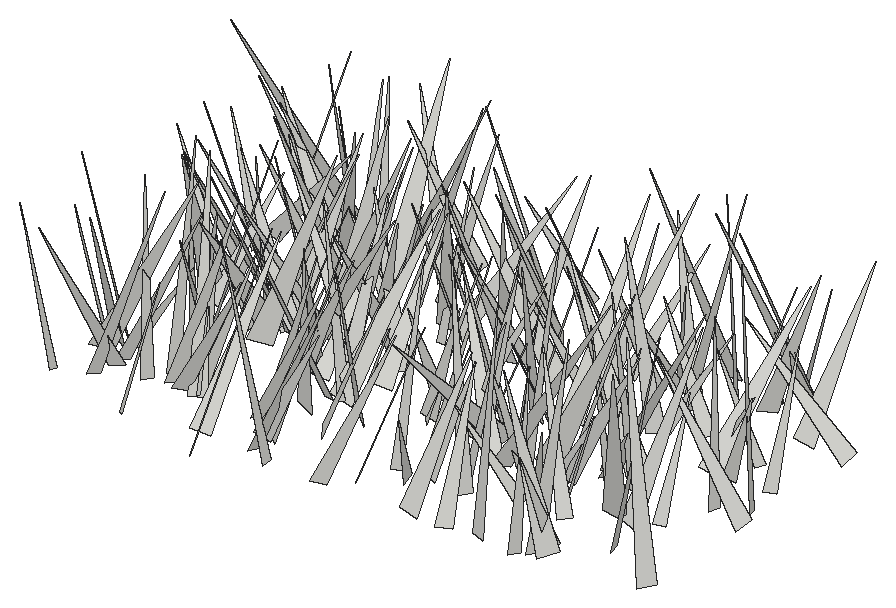
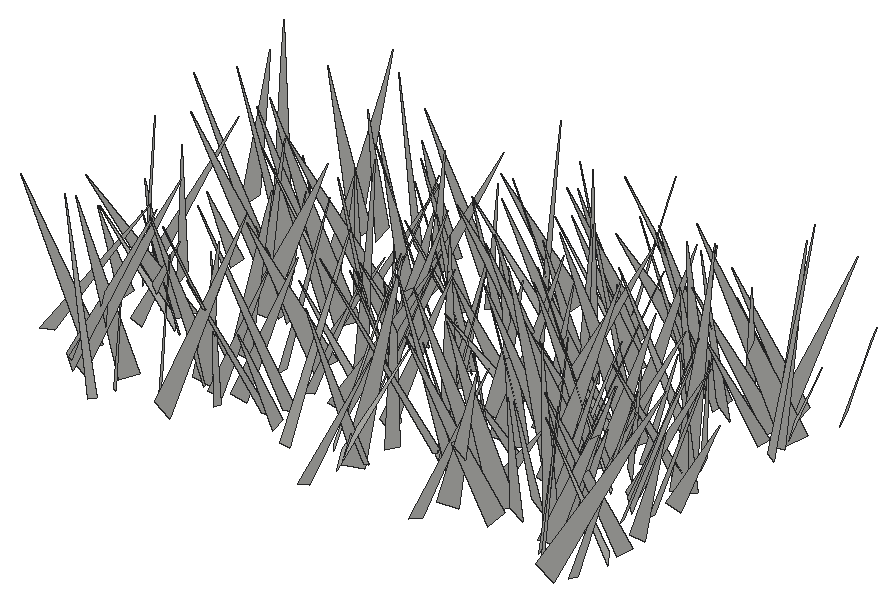
# SketchUp Ruby script. Lengths in inches.
U = 1.inch
M = Sketchup.active_model
def pt(a) = Geom::Point3d.new(a.map { |v| v * U })
def face(e, loops, mat)
  f = e.add_face(loops[0].map { |a| pt(a) })
  loops[1..].each { |l| e.add_face(l.map { |a| pt(a) }).erase! }
  f.material = f.back_material = mat if mat
  f
end
# faces: each face lists its corners as indices into pts; further lists are holes
def faces(e, pts, list, mat = nil) = list.each { |f| face(e, (f[0].is_a?(Array) ? f : [f]).map { |l| l.map { |i| pts[i] } }, mat) }
# xy, xz, yz: faces in a plane at the given z, y or x. An outline is a flat list of corners, or four numbers for a rectangle; further outlines are holes
def ring(l) = l.size == 4 ? [[l[0], l[1]], [l[2], l[1]], [l[2], l[3]], [l[0], l[3]]] : l.each_slice(2).to_a
def flat(e, list, mat, &to3) = list.each { |f| face(e, (f[0].is_a?(Array) ? f : [f]).map { |l| ring(l).map { |u, v| to3.(u, v) } }, mat) }
def xy(e, z, list, mat = nil) = flat(e, list, mat) { |x, y| [x, y, z] }
def xz(e, y, list, mat = nil) = flat(e, list, mat) { |x, z| [x, y, z] }
def yz(e, x, list, mat = nil) = flat(e, list, mat) { |y, z| [x, y, z] }
def lines(e, pts, list) = list.each { |a, b| e.add_line(pt(pts[a]), pt(pts[b])) }
# prism: a flat outline (further loops are holes) pulled along v
def prism(e, loops, v, mat = nil)
  f = face(e, loops, mat); d = Geom::Vector3d.new(v.map { |x| x * U })
  f.pushpull(f.normal.samedirection?(d) ? d.length : -d.length)
end
def box(e, o, s, mat = nil) = prism(e, [[o, [o[0] + s[0], o[1], o[2]], [o[0] + s[0], o[1] + s[1], o[2]], [o[0], o[1] + s[1], o[2]]]], [0, 0, s[2]], mat)
def at(x, y, z, deg = 0) = Geom::Transformation.translation(pt([x, y, z])) * Geom::Transformation.rotation(ORIGIN, Z_AXIS, deg.degrees)
def axes(o, x, y, z) = Geom::Transformation.new([*x, 0, *y, 0, *z, 0, *pt(o).to_a, 1])
def part(name) = M.definitions.add(name)
# library, detail: a bought-in or finely detailed component or shape, given as its bounding box
def library(name, o, s) = part(name).tap { |d| box(d.entities, o, s) }
def detail(e, o, s) = box(e.add_group.entities, o, s)
def put(e, d, t, mat = nil) = e.add_instance(d, t).tap { |i| i.material = mat if mat }
def group(e, t, mat = nil) = e.add_group.tap { |g| g.transformation = t; g.material = mat if mat }.entities
root = M.entities
c1 = part("fur_instance\#9")
p = [[0.8125,0,1.79],[0.67,-0.02,1.48],[0,-0.11,0],[0,0.11,0]]
faces(c1.entities,p,[[0,1,2,3]])
put(root,c1,axes([495.01,358.53,-21.66],[4.68158,-4.31782,3.21331],[-4.18207,-5.59908,-1.43065],[-3.3881,0.94493,6.20597]))
put(root,c1,axes([494.79,359.46,-21.66],[4.08531,-1.79648,1.28746],[-1.24322,-4.1049,-1.78292],[-1.82737,-1.22355,4.09124]))
put(root,c1,axes([473.0625,356.67,-21.66],[-7.26619,-2.16018,0.91047],[-2.32448,7.02333,-1.88745],[0.30351,2.07347,7.34176]))
put(root,c1,axes([468.41,354.61,-21.66],[6.47169,4.71895,0.84374],[4.29058,-6.33416,2.51645],[-2.13805,1.57262,7.60387]))
put(root,c1,axes([461.51,355.93,-21.66],[2.88186,3.44939,0.31018],[3.15851,-2.7832,1.60537],[-1.42067,0.8094,4.19835]))
put(root,c1,axes([457.41,360.6875,-21.66],[0.6668,-6.36542,0.43774],[-6.10772,-0.7641,-1.80742],[-1.84553,0.22889,6.13974]))
put(root,c1,axes([484.39,357.22,-21.66],[0.24671,6.36494,1.6516],[6.30189,0.24313,-1.87833],[1.87786,-1.65213,6.08648]))
put(root,c1,axes([477.34,356.72,-21.66],[5.30796,-1.91017,1.71118],[-2.50762,-4.68997,2.54311],[-0.53734,3.01775,5.03546]))
put(root,c1,axes([470.7,359.16,-21.66],[2.62599,-5.06265,0.78885],[-4.77605,-2.09765,2.43674],[1.85526,1.76578,5.15641]))
put(root,c1,axes([481.65,360.63,-21.66],[4.12034,-0.14152,0.59374],[0.17297,-3.61498,-2.06197],[-0.58535,-2.06437,3.57009]))
put(root,c1,axes([487.48,357.11,-21.66],[-4.32625,3.6169,1.13686],[3.35652,4.45591,-1.40339],[1.76301,0.39209,5.46158]))
put(root,c1,axes([454.46,357.73,-21.66],[-5.41168,-1.42657,0.35166],[-1.45652,5.03228,-1.99993],[-0.1932,2.0214,5.22701]))
put(root,c1,axes([493.19,357.29,-21.66],[-6.05732,0.47074,1.68041],[-0.07648,5.99257,-1.95441],[1.74342,1.89841,5.75265]))
put(root,c1,axes([471.32,357.58,-21.66],[6.28882,0.29269,0.74734],[0.08478,-6.11246,1.68051],[-0.79813,1.65699,6.06719]))
put(root,c1,axes([489.93,357.61,-21.66],[3.45024,7.01244,2.07893],[6.95776,-3.8555,1.45774],[-2.25516,-1.1667,7.67811]))
put(root,c1,axes([494.21,358.21,-21.66],[-6.74927,1.80081,2.69667],[1.18797,7.16726,-1.81295],[3.01723,1.2063,6.74602]))
put(root,c1,axes([462.65,360.75,-21.66],[4.53332,-3.78068,0.06575],[-3.6354,-4.32956,1.69931],[1.04008,1.34544,5.65304]))
put(root,c1,axes([455.38,363.32,-21.66],[-1.80775,-6.68688,0.47497],[-6.40102,1.86794,1.93536],[1.9917,-0.06601,6.65106]))
put(root,c1,axes([467.12,357.18,-21.66],[-4.67484,5.38464,0.57126],[4.73589,4.43174,-3.01759],[2.62527,1.59378,6.46085]))
put(root,c1,axes([479.14,358.47,-21.66],[4.7893,3.01055,0.30481],[2.77693,-4.59952,1.79634],[-1.20208,1.36921,5.36414]))
put(root,c1,axes([489.45,362.83,-21.66],[-4.59032,-0.23962,0.17171],[-0.16134,4.28449,1.66587],[0.24672,-1.65642,4.28408]))
put(root,c1,axes([456.87,358.93,-21.66],[6.5419,0.41912,1.71437],[-0.23349,-6.31856,2.43568],[-1.74935,2.41069,6.08602]))
put(root,c1,axes([502.66,359.23,-21.66],[-8.1921,1.36867,0.61461],[1.20152,8.02801,-1.8625],[0.89853,1.74336,8.09413]))
put(root,c1,axes([463.77,361.33,-21.66],[3.63408,5.21962,1.38175],[5.32326,-3.18476,-1.96987],[0.90365,-2.23003,6.04736]))
put(root,c1,axes([468.93,361.03,-21.66],[5.6454,-1.61471,0.55375],[-1.70236,-5.46688,1.41409],[-0.12614,1.5134,5.69896]))
put(root,c1,axes([482.48,361.83,-21.66],[0.05129,-4.93553,2.34933],[-4.99892,0.90807,2.01684],[2.21125,2.16734,4.50493]))
put(root,c1,axes([468.37,363.05,-21.66],[5.01746,5.30698,2.27397],[5.71554,-4.13917,-2.95123],[0.81705,-3.63499,6.68051]))
put(root,c1,axes([473.91,365.3125,-21.66],[-3.7888,-7.35051,1.42507],[-6.56657,4.02946,3.32556],[3.59735,-0.38635,7.57137]))
put(root,c1,axes([471.67,359.15,-21.66],[4.6203,4.92142,0.32663],[4.69042,-4.52255,1.79463],[-1.52544,1.00021,6.50745]))
put(root,c1,axes([473.32,362.11,-21.66],[5.31801,3.62577,0.57345],[3.65614,-5.14142,-1.39812],[0.32822,-1.47507,6.28273]))
put(root,c1,axes([454.96,364.62,-21.66],[-4.90749,-6.3294,1.61985],[-6.13533,5.16095,1.5783],[2.24565,0.26836,7.85199]))
put(root,c1,axes([495.2,365.25,-21.66],[1.43301,-8.2393,0.15598],[-8.02359,-1.35888,1.93375],[1.87948,0.48092,8.13635]))
put(root,c1,axes([461.71,361.26,-21.66],[6.69974,-1.69034,1.74311],[-2.11177,-6.58131,1.73465],[-1.19837,2.1474,6.68841]))
put(root,c1,axes([470.45,363.9,-21.66],[-1.45623,-6.82166,1.9418],[-6.84757,1.86878,1.42991],[1.84835,1.54881,6.82723]))
put(root,c1,axes([460.1,360.48,-21.66],[-6.71472,0.14595,1.05093],[-0.21339,6.41005,-2.25365],[1.03933,2.25902,6.32691]))
put(root,c1,axes([455.04,361.94,-21.66],[6.5519,-4.81181,0.9912],[-4.80718,-5.93833,2.94799],[1.01342,2.94042,7.57563]))
put(root,c1,axes([464.29,361.04,-21.66],[-5.1152,1.11044,1.16629],[0.73583,5.06638,-1.59654],[1.43244,1.36283,4.98492]))
put(root,c1,axes([489.3,364.63,-21.66],[-0.15941,-4.26775,0.08772],[-3.87813,0.18147,1.78158],[1.78369,0.01316,3.88138]))
put(root,c1,axes([455.64,362.03,-21.66],[-4.45593,-2.02584,0.38216],[-1.95722,3.87117,-2.29973],[-0.64758,2.23951,4.32095]))
put(root,c1,axes([460.95,366,-21.66],[-1.84691,-6.18778,0.26193],[-5.9057,1.84189,1.87043],[1.86547,-0.29517,6.18071]))
put(root,c1,axes([464.13,360.71,-21.66],[0.27633,8.1596,0.76138],[7.93766,-0.45592,2.00518],[-2.0377,-0.66947,7.91421]))
put(root,c1,axes([457.15,361.625,-21.66],[6.04009,-0.71684,0.90558],[-1.00409,-5.64184,2.23115],[-0.57074,2.3393,5.65849]))
put(root,c1,axes([485.76,361.42,-21.66],[-7.72963,0.57294,0.92033],[0.30078,7.49944,-2.14251],[1.04153,2.08628,7.44883]))
put(root,c1,axes([497.92,361.75,-21.66],[6.4621,3.38539,1.99868],[3.00841,-6.73382,1.67909],[-2.53082,0.63956,7.09931]))
put(root,c1,axes([483.41,368.64,-21.66],[5.32765,-5.22538,0.29084],[-4.03169,-4.36253,-4.52625],[-3.33686,-3.07194,5.93309]))
put(root,c1,axes([456.56,363.36,-21.66],[3.29977,-2.51906,0.3221],[-2.3698,-2.86445,1.87534],[0.91296,1.66948,3.70368]))
put(root,c1,axes([480.27,361.18,-21.66],[2.16067,6.65454,0.44246],[6.23565,-2.18071,2.34697],[-2.36543,0.32979,6.59114]))
put(root,c1,axes([461.14,361.86,-21.66],[2.8075,7.47142,1.47372],[7.21104,-3.11318,2.04573],[-2.44844,-0.60171,7.71486]))
put(root,c1,axes([491.26,365.27,-21.66],[3.99613,2.0991,0.80323],[2.24013,-3.58697,-1.77087],[0.18236,-1.93595,4.15203]))
put(root,c1,axes([492.84,362.98,-21.66],[-1.19348,5.65379,0.3473],[5.3271,0.99964,2.033],[-1.92561,-0.73875,5.40894]))
put(root,c1,axes([470.83,365.9,-21.66],[-3.56669,-5.90918,0.59479],[-5.71236,3.22345,-2.22975],[-1.62517,1.63841,6.53207]))
put(root,c1,axes([484.51,363.29,-21.66],[4.61652,6.22378,1.13894],[6.03614,-4.75491,1.51682],[-1.89675,0.0163,7.59914]))
put(root,c1,axes([480.61,363.97,-21.66],[3.00596,2.69315,0.13963],[2.45938,-2.82346,1.51258],[-1.10635,1.04086,3.74179]))
put(root,c1,axes([467.49,368.98,-21.66],[-1.30326,-6.4856,0.41929],[-6.05179,1.36694,2.33336],[2.36951,-0.07596,6.19006]))
put(root,c1,axes([462.64,370.46,-21.66],[6.08431,-4.17162,0.61258],[-3.3903,-5.47976,-3.64343],[-2.50671,-2.71408,6.41457]))
put(root,c1,axes([472.63,367.23,-21.66],[3.70621,1.73352,0.50221],[1.78343,-3.34171,-1.62653],[0.27688,-1.67963,3.75439]))
put(root,c1,axes([489.52,367.13,-21.66],[2.95462,-6.48005,1.02046],[-5.97059,-2.19282,3.36242],[2.71745,2.2277,6.27814]))
put(root,c1,axes([496.72,364.875,-21.66],[1.72672,7.47142,1.23195],[7.48463,-1.49226,-1.44043],[1.14896,-1.50745,7.53186]))
put(root,c1,axes([467.25,367.52,-21.66],[3.81653,-4.78014,0.36891],[-4.62204,-3.54318,1.90641],[1.2738,1.46558,5.81217]))
put(root,c1,axes([482,367.45,-21.66],[1.0853,-7.02468,2.48253],[-7.23303,-0.3918,2.05344],[1.78669,2.68091,6.80495]))
put(root,c1,axes([486.08,366.82,-21.66],[-6.99068,-2.50094,0.47101],[-2.54423,6.83653,-1.46112],[-0.05835,1.53405,7.27938]))
put(root,c1,axes([477.54,367.91,-21.66],[1.22983,-5.08709,1.30795],[-5.046,-0.77126,1.74491],[1.45845,1.62123,4.93419]))
put(root,c1,axes([485.17,365.87,-21.66],[7.21653,-2.33327,0.39687],[-2.31249,-6.67999,2.77668],[0.50399,2.75925,7.05779]))
put(root,c1,axes([480.72,363.98,-21.66],[4.07419,5.57288,0.07978],[5.18286,-3.82462,2.48447],[-2.04971,1.40628,6.44076]))
put(root,c1,axes([484.37,366.11,-21.66],[-3.04335,5.85133,0.32291],[5.70958,2.87864,1.64877],[-1.32023,-1.03909,6.38604]))
put(root,c1,axes([487.54,367.96,-21.66],[4.40599,-6.63506,1.39046],[-6.52465,-3.70025,3.01783],[1.84021,2.76664,7.37085]))
put(root,c1,axes([466.51,368.04,-21.66],[6.17977,-5.38552,0.13557],[-5.06059,-5.73249,2.95646],[1.84733,2.31224,7.64543]))
put(root,c1,axes([477.4,367.84,-21.66],[5.01329,4.55618,1.17415],[4.70331,-4.80639,-1.43108],[0.12753,-1.84671,6.62147]))
put(root,c1,axes([471.96,366.15,-21.66],[-6.70082,0.16595,0.10129],[0.12128,6.29761,-2.29436],[0.15195,2.29157,6.29797]))
put(root,c1,axes([490.59,365.47,-21.66],[4.99959,5.18328,0.38062],[5.01525,-4.9501,1.53324],[-1.36326,0.79826,7.03643]))
put(root,c1,axes([498.22,366.13,-21.66],[-3.90191,2.21296,0.38649],[1.88444,3.64598,-1.85127],[1.22289,1.44261,4.08594]))
put(root,c1,axes([456.65,371.74,-21.66],[7.11754,-4.23376,0.53848],[-3.90576,-6.88369,-2.49681],[-1.7204,-1.88792,7.89621]))
put(root,c1,axes([471.64,366.18,-21.66],[-0.75445,7.6495,1.46212],[7.18414,1.25072,-2.83648],[3.00677,-1.06897,7.14412]))
put(root,c1,axes([502.54,369.54,-21.66],[-6.59727,0.97904,0.29915],[1.02311,6.37288,1.70633],[0.03533,-1.73199,6.44755]))
put(root,c1,axes([476.84,370.16,-21.66],[3.36953,-3.09183,0.80409],[-2.80421,-3.42236,-1.4084],[-1.53048,-0.53643,4.35081]))
put(root,c1,axes([493.36,367.04,-21.66],[-5.59441,-0.96055,0.72122],[-1.15543,5.24244,-1.98041],[0.32833,2.08191,5.31959]))
put(root,c1,axes([460.2,366.45,-21.66],[6.70956,3.50603,1.11128],[3.28027,-6.75003,1.49074],[-1.66343,0.8308,7.42214]))
put(root,c1,axes([460.97,370.38,-21.66],[-3.68775,-0.43694,1.2324],[0.03671,3.65173,1.40455],[1.30705,-1.33536,3.43768]))
put(root,c1,axes([494.14,368.64,-21.66],[1.80379,6.11401,2.80003],[6.29213,-2.55743,1.53087],[-2.37284,-2.13386,6.18799]))
put(root,c1,axes([486.97,366.5,-21.66],[3.53249,6.50702,1.2231],[6.07163,-3.73652,2.34297],[-2.64057,0.11331,7.02355]))
put(root,c1,axes([487.37,369.79,-21.66],[-2.45268,-3.25533,0.28731],[-3.08329,2.18606,-1.55237],[-1.08306,1.14864,3.76868]))
put(root,c1,axes([457.76,368.17,-21.66],[-5.24858,-0.93793,1.2858],[-1.33069,5.01688,-1.77222],[0.87308,2.00792,5.02857]))
put(root,c1,axes([482.15,367.73,-21.66],[3.84867,2.11329,0.22175],[1.92609,-3.66331,1.48248],[-0.8974,1.20066,4.13285]))
put(root,c1,axes([482.04,370.46,-21.66],[-2.37076,-5.83706,1.32394],[-5.9146,2.06646,-1.48049],[-0.91737,1.76156,6.12372]))
put(root,c1,axes([462.75,368.8125,-21.66],[5.54256,-5.39998,2.31392],[-5.86744,-4.92827,2.55329],[0.29519,3.43313,7.30483]))
put(root,c1,axes([464.42,373.07,-21.66],[-5.86145,-3.99032,0.23805],[-3.68658,5.55942,2.41617],[1.54546,-1.87245,6.66644]))
put(root,c1,axes([468.73,367.71,-21.66],[-1.68385,4.77561,0.18208],[4.53538,1.65768,-1.53538],[1.50664,0.34725,4.82539]))
put(root,c1,axes([456.03,371.4,-21.66],[-0.42992,-4.68733,0.89248],[-4.33891,0.75688,1.88505],[1.98531,0.63912,4.31306]))
put(root,c1,axes([491.55,369.12,-21.66],[7.5928,-1.32868,0.07278],[-1.31152,-7.40102,1.71058],[0.22497,1.69728,7.51598]))
put(root,c1,axes([463.15,371.04,-21.66],[-3.41079,-4.86692,0.40111],[-4.72199,3.16213,-1.78467],[-1.24525,1.33989,5.66881]))
put(root,c1,axes([470.875,367.41,-21.66],[-5.5806,3.5391,0.90465],[3.04631,5.42049,-2.4135],[2.01583,1.60617,6.15169]))
put(root,c1,axes([482.93,372.41,-21.66],[-1.97553,-6.78705,1.45707],[-6.65434,2.28292,1.61176],[1.97656,0.90224,6.88251]))
put(root,c1,axes([470.3,373.78,-21.66],[3.62515,-5.36286,0.15908],[-5.03579,-3.46731,-2.13211],[-1.85105,-1.06996,6.11196]))
put(root,c1,axes([484.31,368.57,-21.66],[2.91558,3.30379,0.88214],[2.68077,-2.92801,2.10571],[-2.12289,0.83996,3.8706]))
put(root,c1,axes([469.28,369.57,-21.66],[7.05742,-1.09775,2.22467],[-1.64487,-7.09246,1.71837],[-1.85705,2.1103,6.93249]))
put(root,c1,axes([493.01,370.57,-21.66],[-4.31341,6.46311,1.11663],[6.32564,3.74609,2.75266],[-1.73345,-2.41229,7.26637]))
put(root,c1,axes([464.99,368.66,-21.66],[4.59925,2.87418,0.36346],[2.61006,-4.40682,1.82035],[-1.25721,1.36572,5.10885]))
put(root,c1,axes([490.875,369.68,-21.66],[4.03542,0.28371,1.50858],[-0.2798,-4.0361,1.5075],[-1.50932,1.50677,3.754]))
put(root,c1,axes([463.28,371.47,-21.66],[-4.72001,4.32069,1.36462],[4.52973,4.45158,1.57294],[-0.11027,-2.07946,6.20264]))
put(root,c1,axes([499.73,369.97,-21.66],[-6.28866,-0.36775,1.68536],[-0.82762,6.23312,-1.72806],[1.51351,1.8804,6.05775]))
put(root,c1,axes([472.62,369.21,-21.66],[-1.93845,6.02083,0.54238],[5.77969,2.01278,-1.68701],[1.77192,0.02133,6.09606]))
put(root,c1,axes([468.76,371.22,-21.66],[-3.29072,5.65648,0.59206],[5.32719,2.82602,2.60955],[-1.99181,-1.7869,6.00123]))
put(root,c1,axes([468.65,373.71,-21.66],[1.7793,-6.50243,0.4842],[-6.28195,-1.575,1.93351],[1.74732,0.95904,6.45825]))
put(root,c1,axes([472.44,371.65,-21.66],[-2.33709,5.71521,1.48586],[5.84354,2.00796,1.46781],[-0.85111,-1.90732,5.99759]))
put(root,c1,axes([468.56,373.19,-21.66],[3.57739,2.98141,0.96801],[3.07785,-3.06266,-1.94177],[0.59384,-2.08684,4.23274]))
put(root,c1,axes([471.87,369.36,-21.66],[4.84887,3.21318,0.05137],[2.84684,-4.33809,2.62966],[-1.49084,2.16682,5.18854]))
put(root,c1,axes([457.1,371.06,-21.66],[0.04423,5.29855,0.55334],[5.02486,0.14232,-1.76445],[1.76963,-0.53655,4.99632]))
put(root,c1,axes([465.27,371.98,-21.66],[-5.24793,-3.08562,0.82091],[-3.15493,4.76816,-2.24651],[-0.49124,2.34081,5.65818]))
put(root,c1,axes([497.93,373.73,-21.66],[1.41621,-4.16021,0.5332],[-4.01988,-1.18575,1.42542],[1.19673,0.94019,4.15706]))
put(root,c1,axes([458.76,374.5,-21.66],[-2.19806,-5.17129,0.07017],[-4.98418,2.09779,-1.52836],[-1.38027,0.66005,5.4072]))
put(root,c1,axes([460.77,372.03,-21.66],[2.36274,4.29484,1.97791],[3.91667,-3.01643,1.87116],[-2.64906,-0.62918,4.53067]))
put(root,c1,axes([501.89,371.14,-21.66],[-7.32928,-2.99407,2.48715],[-3.76161,6.81126,-2.88543],[1.00033,3.67572,7.37273]))
put(root,c1,axes([456.2,375.48,-21.66],[-5.34659,-1.99732,0.9572],[-1.60106,5.21354,1.93576],[1.5304,-1.52357,5.36919]))
put(root,c1,axes([465.65,371.77,-21.66],[7.81962,-2.04899,1.63917],[-2.46618,-7.49875,2.3913],[-0.8962,2.75717,7.72182]))
put(root,c1,axes([462.74,372.47,-21.66],[-0.40245,7.17423,1.83924],[7.10701,0.89237,-1.92572],[2.08393,-1.65784,6.92265]))
put(root,c1,axes([486.96,375.49,-21.66],[-5.96376,-1.66281,1.60864],[-1.32131,6.09893,1.40577],[1.89916,-0.97833,6.02952]))
put(root,c1,axes([460.3,374.58,-21.66],[6.41393,4.45568,0.74677],[4.39818,-5.86174,-2.80093],[1.0328,-2.70854,7.29015]))
put(root,c1,axes([457.24,377.24,-21.66],[-5.6995,-3.45113,0.56108],[-3.05969,5.44221,2.39374],[1.69215,-1.78365,6.21808]))
put(root,c1,axes([477.57,374.12,-21.66],[2.82226,4.09729,0.68802],[3.94816,-2.38599,-1.98631],[1.29353,-1.65697,4.56152]))
put(root,c1,axes([464.25,376.36,-21.66],[-0.98604,-7.77609,1.14314],[-7.75331,0.77346,-1.42635],[-1.28859,1.29646,7.70749]))
put(root,c1,axes([476.89,376.17,-21.66],[4.69242,0.16576,0.10905],[0.19618,-4.2622,-1.96297],[-0.02968,-1.96577,4.26532]))
put(root,c1,axes([455.8,373.73,-21.66],[-1.87407,5.07403,0.37598],[4.58214,1.50899,2.47512],[-2.21159,-1.17322,4.80954]))
put(root,c1,axes([478.56,377.34,-21.66],[-5.31145,-3.30369,0.30508],[-3.10318,5.15062,1.7494],[1.17379,-1.33255,6.00546]))
put(root,c1,axes([495.26,375.85,-21.66],[3.7363,2.07589,0.22504],[1.88074,-3.14536,-2.2112],[0.90706,-2.02911,3.65784]))
put(root,c1,axes([466.17,373.06,-21.66],[6.99612,0.8962,1.32294],[0.53893,-6.91662,1.83548],[-1.5043,1.69005,6.81028]))
put(root,c1,axes([458.17,375.3,-21.66],[-4.54723,-4.75664,0.92618],[-4.80738,4.26788,-1.68375],[-0.61038,1.82216,6.36144]))
put(root,c1,axes([483.75,376.63,-21.66],[-4.12735,0.23871,1.0618],[0.66209,3.85593,1.70672],[0.86374,-1.81501,3.76552]))
put(root,c1,axes([471.13,377.94,-21.66],[1.38948,-7.3294,0.52561],[-7.22169,-1.26322,1.47599],[1.35779,0.7818,7.31247]))
put(root,c1,axes([490.44,375.49,-21.66],[0.55965,-6.1533,3.26603],[-6.71098,-1.35523,-1.40332],[-1.86889,3.02383,6.01722]))
put(root,c1,axes([472.05,378.1,-21.66],[-4.28945,-4.51982,0.83876],[-4.25056,4.33652,1.63064],[1.75072,-0.54543,6.01408]))
put(root,c1,axes([464.37,375.34,-21.66],[-0.74897,7.24815,2.93985],[7.55595,1.43371,-1.60981],[2.0214,-2.6736,7.1067]))
put(root,c1,axes([501.15,373.97,-21.66],[-4.3486,2.21974,0.80785],[1.83051,4.23636,-1.78683],[1.49303,1.27131,4.54366]))
put(root,c1,axes([477.14,376.97,-21.66],[-2.01567,-6.30283,1.43527],[-6.28052,1.55369,-1.99742],[-1.52993,1.92587,6.30864]))
put(root,c1,axes([498.44,376.35,-21.66],[-0.27177,-3.75184,1.87256],[-3.70908,-0.66019,-1.86105],[-1.95589,1.77327,3.26904]))
put(root,c1,axes([462.15,377.99,-21.66],[-4.28655,1.17606,1.86698],[1.8295,4.17484,1.57066],[1.23356,-2.10497,4.15821]))
put(root,c1,axes([481.04,377.07,-21.66],[-4.16636,5.9481,1.52453],[5.74666,3.12806,3.50054],[-2.16332,-3.14611,6.36276]))
put(root,c1,axes([496.4375,373.62,-21.66],[-2.65177,6.66161,0.65253],[5.97681,2.67255,-2.995],[3.01341,0.56142,6.51452]))
put(root,c1,axes([490.56,376.5,-21.66],[2.95433,4.07724,0.35212],[3.82019,-2.59183,-2.04072],[1.46767,-1.46099,4.60298]))
put(root,c1,axes([485.14,373.26,-21.66],[-5.76444,5.45156,1.05869],[4.71185,5.60881,-3.22628],[2.93919,1.70025,7.24841]))
put(root,c1,axes([475,378.99,-21.66],[6.59264,-0.88288,1.14982],[-0.53637,-6.4595,-1.88457],[-1.3468,-1.74924,6.37893]))
put(root,c1,axes([481.52,374.27,-21.66],[4.88269,3.53574,0.69101],[3.04894,-4.67553,2.3797],[-1.91908,1.56767,5.53887]))
put(root,c1,axes([467.67,375.03,-21.66],[3.89032,1.8987,0.46131],[1.51623,-3.58179,1.95558],[-1.23244,1.58688,3.86204]))
put(root,c1,axes([493.38,377.36,-21.66],[-3.16425,3.77948,0.90882],[3.82647,2.82214,1.58634],[-0.68447,-1.69527,4.66695]))
put(root,c1,axes([467.05,377.17,-21.66],[-1.66623,3.3763,0.05798],[2.90925,1.40249,1.93607],[-1.71436,-0.9015,3.22914]))
put(root,c1,axes([496.47,374.89,-21.66],[4.76717,4.34009,0.09976],[4.0907,-4.54047,2.05487],[-1.45344,1.45601,6.11063]))
put(root,c1,axes([458.59,379.84,-21.66],[0.69444,-4.60057,1.02449],[-4.36557,-1.0182,-1.61314],[-1.77671,0.70364,4.36409]))
put(root,c1,axes([488.49,380.63,-21.66],[1.56687,-4.2825,0.24372],[-4.04586,-1.5617,-1.43053],[-1.42486,-0.27491,4.32996]))
put(root,c1,axes([472.04,376.07,-21.66],[2.45384,5.3856,0.3895],[5.06414,-2.44383,1.88676],[-1.87372,0.44803,5.60947]))
put(root,c1,axes([478,381.37,-21.66],[-5.39374,-4.42373,0.73063],[-4.15874,5.36317,1.77113],[1.67573,-0.92879,6.74722]))
put(root,c1,axes([465.64,379.72,-21.66],[3.73133,2.74864,1.27928],[3.02044,-3.19509,-1.94493],[0.26177,-2.31318,4.20655]))
put(root,c1,axes([455.11,378.33,-21.66],[-1.60239,4.56784,1.22355],[4.62571,1.24567,1.40748],[-0.98238,-1.58525,4.63161]))
put(root,c1,axes([486.93,380.09,-21.66],[0.61294,-5.47928,1.38132],[-5.30961,-1.0339,-1.7451],[-1.93355,1.10218,5.22999]))
put(root,c1,axes([502.45,380.66,-21.66],[-5.96221,1.49508,0.02596],[1.36332,5.39133,2.61894],[-0.61423,-2.54602,5.56097]))
put(root,c1,axes([472.27,377.69,-21.66],[3.56611,7.00423,0.23479],[6.50816,-3.2121,-3.02618],[2.59966,-1.56674,7.25387]))
put(root,c1,axes([460,378.89,-21.66],[-2.19401,4.08598,0.64459],[3.98986,1.89782,1.55038],[-1.09165,-1.27572,4.37096]))
put(root,c1,axes([480.73,383.0625,-21.66],[-3.5223,-6.70382,0.02091],[-6.50166,3.42181,1.83516],[1.63401,-0.83562,7.34711]))
put(root,c1,axes([454.53,380.36,-21.66],[2.58062,-5.27777,0.62862],[-4.46822,-1.77579,3.43383],[2.87837,1.97518,4.76689]))
put(root,c1,axes([459.5,381.79,-21.66],[6.23542,-1.61716,0.46655],[-1.48447,-6.12774,-1.40019],[-0.79324,-1.24458,6.2877]))
put(root,c1,axes([475.46,382.53,-21.66],[5.45366,-4.66647,1.60556],[-4.21255,-5.64853,-2.10822],[-2.57063,-0.64365,6.86103]))
put(root,c1,axes([459.94,380.3125,-21.66],[-5.34119,3.3335,0.99515],[3.47843,5.14626,1.43085],[0.05516,-1.74201,6.13133]))
put(root,c1,axes([469.27,379.75,-21.66],[2.86437,6.58912,2.04567],[6.83224,-2.40073,-1.83379],[0.96006,-2.57407,6.94682]))
put(root,c1,axes([467.7,378.51,-21.66],[7.57177,-0.43303,1.80554],[-0.88332,-7.50835,1.90355],[-1.63317,2.05334,7.34137]))
put(root,c1,axes([487.44,381.67,-21.66],[4.97524,0.71585,1.07536],[1.04452,-4.74693,-1.67259],[-0.76015,-1.83742,4.74004]))
put(root,c1,axes([483.26,379.27,-21.66],[2.59444,7.48207,1.23534],[7.31718,-2.12705,-2.48457],[1.99156,-1.93206,7.51927]))
put(root,c1,axes([459.28,382.53,-21.66],[3.15853,-4.87453,2.05329],[-4.28659,-3.76007,-2.33247],[-3.09874,0.23284,5.31949]))
put(root,c1,axes([490.16,379.81,-21.66],[-1.21025,6.4146,1.42422],[6.45546,0.89059,1.47445],[-1.22575,-1.64315,6.35907]))
put(root,c1,axes([490.11,379.0625,-21.66],[7.12046,1.58475,2.39098],[0.70942,-7.17277,2.64146],[-2.77938,2.22916,6.79964]))
put(root,c1,axes([497.89,383.27,-21.66],[-2.49506,-7.82927,1.12782],[-7.54738,2.00233,-2.79687],[-2.3678,1.86761,7.7266]))
put(root,c1,axes([459.04,383.45,-21.66],[6.14406,2.36607,3.59044],[3.36505,-6.54408,-1.44586],[-2.67694,-2.79567,6.42319]))
put(root,c1,axes([484.18,380.59,-21.66],[1.81357,5.35205,0.20733],[5.12174,-1.66889,-1.72019],[1.56691,-0.73948,5.38279]))
put(root,c1,axes([462.77,379.09,-21.66],[1.87355,6.48838,0.26131],[6.01197,-1.83596,2.48253],[-2.45429,0.45575,6.28063]))
put(root,c1,axes([498.75,380.48,-21.66],[-0.63507,6.95916,1.46669],[6.78735,1.03289,-1.962],[2.12438,-1.21968,6.70699]))
put(root,c1,axes([494.3,382.28,-21.66],[5.13759,-3.83835,0.8309],[-3.9202,-4.93031,1.46363],[0.23526,1.66651,6.24384]))
put(root,c1,axes([498.59,383.12,-21.66],[-4.44374,-5.75342,0.61079],[-5.6055,4.0905,-2.25122],[-1.43294,1.84058,6.91236]))
put(root,c1,axes([455.02,385.09,-21.66],[-6.16239,-2.08969,1.53365],[-1.42213,6.03269,2.50561],[2.16712,-1.98337,6.00531]))
put(root,c1,axes([464.27,380.7,-21.66],[-3.17908,7.18759,1.82609],[7.05927,3.54175,-1.65087],[2.27218,-0.9472,7.68392]))
put(root,c1,axes([475.26,381.92,-21.66],[0.44188,5.84269,1.52194],[5.83939,-0.02571,-1.59672],[1.53457,-1.58458,5.63763]))
put(root,c1,axes([493.96,384.23,-21.66],[-2.04339,-2.88899,0.9747],[-2.5158,2.26047,1.42575],[1.7225,-0.12566,3.23866]))
put(root,c1,axes([489.81,384.43,-21.66],[-2.55131,-7.67351,1.38924],[-7.65133,2.18082,-2.00574],[-1.50657,1.91917,7.83383]))
put(root,c1,axes([463.2,380.84,-21.66],[1.09357,6.43106,0.77169],[6.11568,-1.28298,2.02542],[-2.13365,-0.38127,6.20097]))
put(root,c1,axes([482.73,381.25,-21.66],[-4.41851,1.16155,1.66424],[0.34777,4.36157,-2.12081],[1.99949,1.8082,4.04655]))
put(root,c1,axes([463.74,382.2,-21.66],[7.28902,-0.71217,0.57332],[-0.83779,-7.04721,1.89755],[-0.36604,1.94818,7.07364]))
put(root,c1,axes([456.89,385.76,-21.66],[-1.39061,-8.04384,0.83594],[-7.45661,0.94696,-3.29214],[-3.13068,1.31752,7.46987]))
put(root,c1,axes([457.53,385.22,-21.66],[-3.39488,-3.98848,1.56761],[-3.7052,3.73666,1.48306],[2.15333,0.14147,5.02331]))
put(root,c1,axes([476.7,382.42,-21.66],[-6.97142,-3.26118,0.0354],[-2.96258,6.29742,-3.28677],[-1.3637,2.99072,6.9594]))
put(root,c1,axes([468.02,385.27,-21.66],[-6.07615,0.58264,0.90457],[0.83184,5.83413,1.82981],[0.68247,-1.92372,5.8233]))
put(root,c1,axes([467.43,382.67,-21.66],[-3.01404,5.97197,0.86388],[5.95256,2.78442,1.51964],[-0.98886,-1.44144,6.51457]))
put(root,c1,axes([494.42,385.98,-21.66],[6.71484,1.18998,0.43364],[1.2609,-6.06064,-2.89345],[0.11927,-2.92333,6.1752]))
put(root,c1,axes([454.84,381.67,-21.66],[5.18703,3.91751,0.7095],[3.72248,-5.18551,1.41748],[-1.41191,0.72053,6.34373]))
put(root,c1,axes([491.78,382.22,-21.66],[-6.04222,-2.58238,2.07365],[-3.21518,5.60869,-2.38377],[0.79453,3.05796,6.1233]))
put(root,c1,axes([476.49,386.3125,-21.66],[-4.86866,0.51762,1.11395],[0.97098,4.41082,2.19421],[0.75234,-2.34296,4.3769]))
